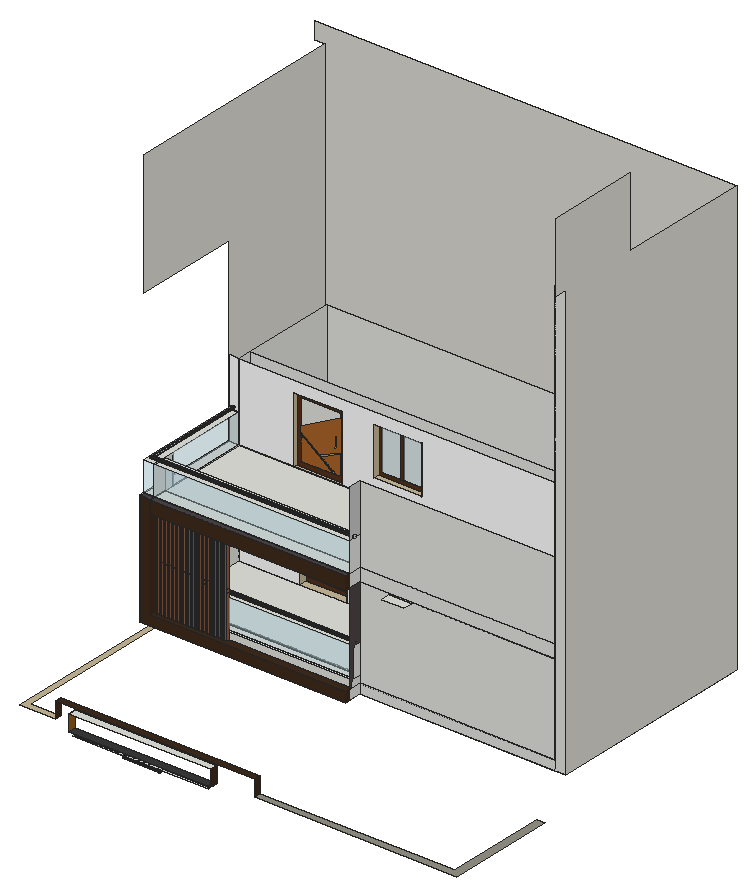
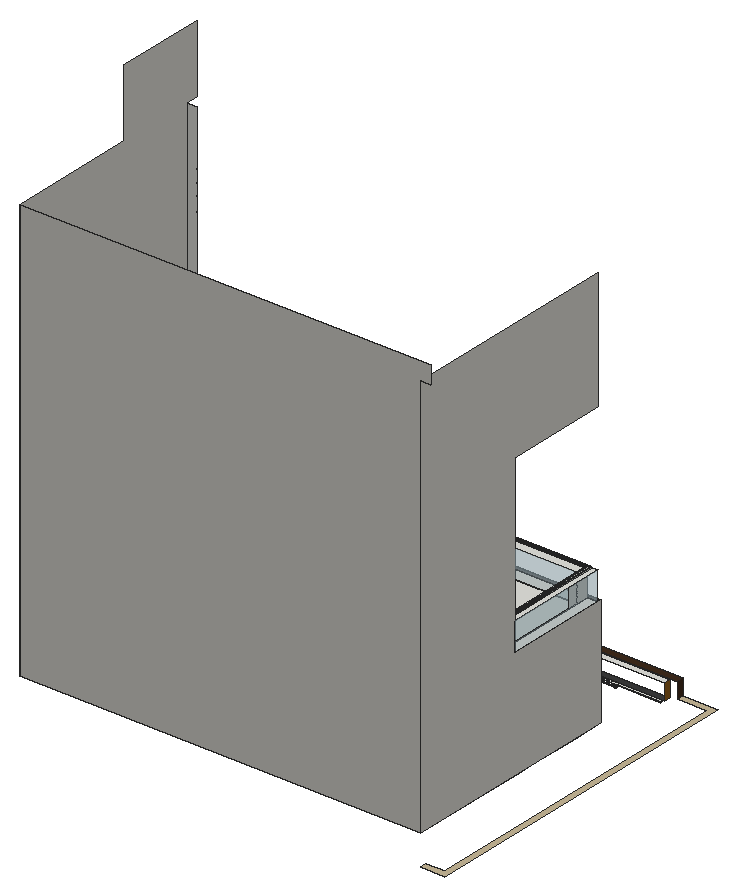
# SketchUp Ruby script. Lengths in inches.
U = 1.inch
M = Sketchup.active_model
def pt(a) = Geom::Point3d.new(a.map { |v| v * U })
def face(e, loops, mat)
  f = e.add_face(loops[0].map { |a| pt(a) })
  loops[1..].each { |l| e.add_face(l.map { |a| pt(a) }).erase! }
  f.material = f.back_material = mat if mat
  f
end
# faces: each face lists its corners as indices into pts; further lists are holes
def faces(e, pts, list, mat = nil) = list.each { |f| face(e, (f[0].is_a?(Array) ? f : [f]).map { |l| l.map { |i| pts[i] } }, mat) }
# xy, xz, yz: faces in a plane at the given z, y or x. An outline is a flat list of corners, or four numbers for a rectangle; further outlines are holes
def ring(l) = l.size == 4 ? [[l[0], l[1]], [l[2], l[1]], [l[2], l[3]], [l[0], l[3]]] : l.each_slice(2).to_a
def flat(e, list, mat, &to3) = list.each { |f| face(e, (f[0].is_a?(Array) ? f : [f]).map { |l| ring(l).map { |u, v| to3.(u, v) } }, mat) }
def xy(e, z, list, mat = nil) = flat(e, list, mat) { |x, y| [x, y, z] }
def xz(e, y, list, mat = nil) = flat(e, list, mat) { |x, z| [x, y, z] }
def yz(e, x, list, mat = nil) = flat(e, list, mat) { |y, z| [x, y, z] }
def lines(e, pts, list) = list.each { |a, b| e.add_line(pt(pts[a]), pt(pts[b])) }
# prism: a flat outline (further loops are holes) pulled along v
def prism(e, loops, v, mat = nil)
  f = face(e, loops, mat); d = Geom::Vector3d.new(v.map { |x| x * U })
  f.pushpull(f.normal.samedirection?(d) ? d.length : -d.length)
end
def box(e, o, s, mat = nil) = prism(e, [[o, [o[0] + s[0], o[1], o[2]], [o[0] + s[0], o[1] + s[1], o[2]], [o[0], o[1] + s[1], o[2]]]], [0, 0, s[2]], mat)
def at(x, y, z, deg = 0) = Geom::Transformation.translation(pt([x, y, z])) * Geom::Transformation.rotation(ORIGIN, Z_AXIS, deg.degrees)
def axes(o, x, y, z) = Geom::Transformation.new([*x, 0, *y, 0, *z, 0, *pt(o).to_a, 1])
def part(name) = M.definitions.add(name)
# library, detail: a bought-in or finely detailed component or shape, given as its bounding box
def library(name, o, s) = part(name).tap { |d| box(d.entities, o, s) }
def detail(e, o, s) = box(e.add_group.entities, o, s)
def put(e, d, t, mat = nil) = e.add_instance(d, t).tap { |i| i.material = mat if mat }
def group(e, t, mat = nil) = e.add_group.tap { |g| g.transformation = t; g.material = mat if mat }.entities
root = M.entities
M.materials.add("[Asphalt New]").color = [76, 68, 70]
M.materials.add("[Blinds Weave]").color = [141, 91, 25]
M.materials.add("[Carrera Marble]").color = [252, 252, 252]
M.materials.add("[Carrera Marble]1").color = [247, 247, 247]
M.materials.add("[Color M02]").color = [198, 198, 198]
M.materials.add("[Color M07]").color = [58, 58, 58]
M.materials.add("[Formica Graystone]1").color = [149, 146, 135]
M.materials.add("[Formica Speckled Grey]").color = [94, 105, 111]
M.materials.add("[Quartz Light Brown]").color = [199, 184, 152]
M.materials.add("[Quartz Light Grey]").color = [251, 251, 252]
M.materials.add("[Sandstone]").color = [63, 43, 28]
M.materials.add("[Terrazzo Tile Light]").color = [219, 217, 210]
M.materials.add("[Translucent Glass Safety]").color = [213, 245, 255]
M.materials["[Translucent Glass Safety]"].alpha = 0.35
M.materials.add("[Wood Bamboo]").color = [168, 99, 40]
M.materials.add("[Wood Floor Light]").color = [181, 156, 112]
M.materials.add("[Wood Veneer 01]").color = [84, 49, 25]
M.materials.add("[Wood Veneer 01]1").color = [120, 70, 37]
M.materials.add("[Wood Veneer 02]").color = [140, 94, 67]
xy(root,91.34,[[140.74,279.21,201.14,281.7],[201.14,279.21,204.61,288.34],[204.61,279.21,225.67,288.34],[229.25,279.21,232.82,288.34],[232.82,279.21,253.76,288.34],
  [253.76,279.21,256.89,288.34],[256.89,279.21,321.11,281.7],[140.74,281.7,201.14,286.88],[256.89,281.7,321.11,286.72],[256.89,286.72,321.11,288.34],
  [140.74,286.88,201.14,288.34]])
xy(root,94.91,[[136.3,279.21,319.42,288.34],[319.42,279.21,324.42,288.34]],"[Color M07]")
xy(root,103.14,[[381.67,279.21,649.65,279.21,649.65,424.96,639.83,424.96,639.83,288.34,381.67,288.34]],"[Formica Graystone]1")
xy(root,103.14,[[71.32,279.21,118.15,279.21,118.15,288.34,78.57,288.34,78.57,734.15,104.01,734.15,104.01,742.77,71.32,742.77]],"[Quartz Light Brown]")
xy(root,116.23,[[136.3,279.21,324.42,288.34]])
xy(root,124.77,[[118.15,279.21,324.42,288.34],[324.42,279.21,381.67,288.34]],"[Sandstone]")
xy(root,144.48,[[635.51,460.01,649.65,725.53],[104.01,479.96,118.15,505.27],[104.01,546.4,118.15,571.71],[104.01,614.47,118.15,639.78],[104.01,670,118.15,695.31],
  [104.01,725.53,118.15,742.77],[118.15,725.53,649.65,742.77]])
xy(root,144.48,[[104.01,436.33,104.01,479.96,118.15,479.96,118.15,505.27,104.01,505.27,104.01,546.4,118.15,546.4,118.15,571.71,104.01,571.71,104.01,614.47,118.15,614.47,118.15,639.78,104.01,639.78,104.01,670,118.15,670,118.15,695.31,104.01,695.31,104.01,725.53,635.51,725.53,635.51,460.01,376.83,460.01,376.83,436.33]],"[Carrera Marble]1")
xy(root,157.48,[[120.21,442.77,123.03,446.4],[125.53,442.77,128.34,446.4],[130.84,442.77,133.65,446.4],[136.15,442.77,138.96,446.4],[141.46,442.77,144.28,446.4],
  [146.78,442.77,149.59,446.4],[151.71,442.77,154.53,446.4],[156.65,442.77,159.46,446.4],[161.59,442.77,164.4,446.4],[166.53,442.77,169.34,446.4],
  [171.46,442.77,174.28,446.4],[176.4,442.77,179.21,446.4],[181.34,442.77,184.15,446.4],[186.28,442.77,189.09,446.4],[191.21,442.77,194.03,446.4],
  [196.15,442.77,198.96,446.4],[201.09,442.77,203.9,446.4],[206.03,442.77,208.84,446.4],[210.96,442.77,213.78,446.4],[118.15,447,376.83,460.01],
  [118.15,460.01,635.5,474.16],[118.15,474.16,635.5,583.41],[118.15,583.41,118.15,601.39,635.5,601.39,635.5,583.41,261.36,583.41,261.36,593.72,198.43,593.72,198.43,583.41],[118.15,601.39,635.5,728.625]])
xy(root,157.48,[[198.43,583.41,261.36,593.72]],"[Quartz Light Brown]")
xy(root,157.48,[[[118.15,436.33,376.83,447],[210.96,442.77,213.78,446.4],[206.03,442.77,208.84,446.4],[201.09,442.77,203.9,446.4],[196.15,442.77,198.96,446.4],[191.21,442.77,194.03,446.4],[186.28,442.77,189.09,446.4],[181.34,442.77,184.15,446.4],[176.4,442.77,179.21,446.4],[171.46,442.77,174.28,446.4],[166.53,442.77,169.34,446.4],[161.59,442.77,164.4,446.4],[156.65,442.77,159.46,446.4],[151.71,442.77,154.53,446.4],[146.78,442.77,149.59,446.4],[141.46,442.77,144.28,446.4],[136.15,442.77,138.96,446.4],[130.84,442.77,133.65,446.4],[125.53,442.77,128.34,446.4],[120.21,442.77,123.03,446.4]]],"[Sandstone]")
xy(root,166.35,[[118.15,449.94,376.83,460.01]])
xy(root,166.35,[[118.15,447,376.83,449.94]],"[Quartz Light Grey]")
xy(root,185.49,[[297.75,583.41,366.57,591.78]],"[Quartz Light Brown]")
xy(root,205.54,[[118.15,449.94,376.83,460.01]])
xy(root,259.32,[[198.43,583.41,261.36,593.72]],"[Quartz Light Brown]")
xy(root,261.87,[[297.75,583.41,366.57,591.78]],"[Quartz Light Brown]")
xy(root,277.48,[[118.15,583.41,635.5,601.39],[118.15,601.39,635.5,728.625]])
xy(root,277.48,[[[118.15,436.33,118.15,583.41,635.5,583.41,635.5,460.01,376.83,460.01,376.83,436.33],[151.71,442.77,154.53,446.4],[166.53,442.77,169.34,446.4],[176.4,442.77,179.21,446.4],[191.21,442.77,194.03,446.4],[201.09,442.77,203.9,446.4],[206.03,442.77,208.84,446.4],[210.96,442.77,213.78,446.4],[196.15,442.77,198.96,446.4],[186.28,442.77,189.09,446.4],[171.46,442.77,174.28,446.4],[181.34,442.77,184.15,446.4],[161.59,442.77,164.4,446.4],[156.65,442.77,159.46,446.4],[146.78,442.77,149.59,446.4],[141.46,442.77,144.28,446.4],[136.15,442.77,138.96,446.4],[125.53,442.77,128.34,446.4],[130.84,442.77,133.65,446.4],[120.21,442.77,123.03,446.4]]],"[Wood Veneer 01]1")
xy(root,278.96,[[419.27,442.77,449.02,455.21]])
xy(root,294.73,[[104.01,442.77,118.15,583.41],[118.15,442.77,376.83,460.01],[118.15,460.01,635.5,583.41],[118.15,583.41,118.15,601.39,635.5,601.39,635.5,583.41,253.72,583.41,253.72,588.28,190.84,588.28,190.84,583.41],[118.15,601.39,635.5,728.625]])
xy(root,294.73,[[104.01,436.33,118.15,442.77],[118.15,436.33,376.83,442.77]],"[Asphalt New]")
xy(root,294.73,[[190.84,583.41,253.72,588.28]],"[Quartz Light Brown]")
xy(root,318.08,[[295.95,583.41,360.57,591.84]],"[Quartz Light Brown]")
xy(root,333.73,[[104.01,442.77,118.15,583.41],[118.15,442.77,376.83,460.01]])
xz(root,436.33,[[104.01,144.48,376.83,144.48,376.83,157.48,118.15,157.48,118.15,294.73,104.01,294.73],[118.15,277.48,376.83,294.73]],"[Sandstone]")
xz(root,442.77,[[104.01,294.73,118.15,333.73],[118.15,294.73,376.83,333.73]],"[Translucent Glass Safety]")
xz(root,442.77,[[120.21,157.48,123.03,277.48],[125.53,157.48,128.34,277.48],[130.84,157.48,133.65,277.48],[136.15,157.48,138.96,277.48],[141.46,157.48,144.28,277.48],
  [146.78,157.48,149.59,277.48],[151.71,157.48,154.53,277.48],[156.65,157.48,159.46,277.48],[161.59,157.48,164.4,277.48],[166.53,157.48,169.34,277.48],
  [171.46,157.48,174.28,277.48],[176.4,157.48,179.21,277.48],[181.34,157.48,184.15,277.48],[186.28,157.48,189.09,277.48],[191.21,157.48,194.03,277.48],
  [196.15,157.48,198.96,277.48],[201.09,157.48,203.9,277.48],[206.03,157.48,208.84,277.48],[210.96,157.48,213.78,277.48]],"[Wood Veneer 02]")
xz(root,446.4,[[120.21,157.48,123.03,277.48],[125.53,157.48,128.34,277.48],[130.84,157.48,133.65,277.48],[136.15,157.48,138.96,277.48],[141.46,157.48,144.28,277.48],
  [146.78,157.48,149.59,277.48],[151.71,157.48,154.53,277.48],[156.65,157.48,159.46,277.48],[161.59,157.48,164.4,277.48],[166.53,157.48,169.34,277.48],
  [171.46,157.48,174.28,277.48],[176.4,157.48,179.21,277.48],[181.34,157.48,184.15,277.48],[186.28,157.48,189.09,277.48],[191.21,157.48,194.03,277.48],
  [196.15,157.48,198.96,277.48],[201.09,157.48,203.9,277.48],[206.03,157.48,208.84,277.48],[210.96,157.48,213.78,277.48]])
xz(root,447,[[118.15,157.48,376.83,166.35]])
xz(root,449.94,[[118.15,166.35,376.83,205.54]],"[Translucent Glass Safety]")
xz(root,460.01,[[376.83,144.48,376.83,157.48,635.5,157.48,635.5,719.42,635.51,719.42,635.51,144.48],[635.51,144.48,649.65,719.42],[118.15,157.48,376.83,166.35],[376.83,157.48,635.5,277.48],[376.83,277.48,635.5,294.73],
  [376.83,294.73,635.5,397.48]])
xz(root,460.01,[[118.15,166.35,376.83,205.54],[118.15,294.73,376.83,333.73]],"[Translucent Glass Safety]")
xz(root,583.41,[[118.15,277.48,635.5,294.73],[104.01,294.73,118.15,333.73],[110.36,335.3,109.91,335.36,109.49,335.54,109.125,335.82,108.85,336.18,108.67,336.6,108.61,337.05,108.67,337.51,108.85,337.93,109.125,338.29,109.49,338.57,109.91,338.74,110.36,338.8,110.82,338.74,111.24,338.57,111.6,338.29,111.88,337.93,112.05,337.51,112.11,337.05,112.05,336.6,111.88,336.18,111.6,335.82,111.24,335.54,110.82,335.36]])
xz(root,583.41,[[[118.15,157.48,198.43,157.48,198.43,259.32,261.36,259.32,261.36,157.48,635.5,157.48,635.5,277.48,118.15,277.48],[297.75,185.49,366.57,261.87]],[[118.15,294.73,190.84,294.73,190.84,382.42,253.72,382.42,253.72,294.73,635.5,294.73,635.5,397.48,118.15,397.48],[295.95,318.08,360.57,382.71]],[[104.01,333.73,118.15,397.48],[110.36,335.3,109.91,335.36,109.49,335.54,109.125,335.82,108.85,336.18,108.67,336.6,108.61,337.05,108.67,337.51,108.85,337.93,109.125,338.29,109.49,338.57,109.91,338.74,110.36,338.8,110.82,338.74,111.24,338.57,111.6,338.29,111.88,337.93,112.05,337.51,112.11,337.05,112.05,336.6,111.88,336.18,111.6,335.82,111.24,335.54,110.82,335.36]]],"[Carrera Marble]")
xz(root,588.28,[[196.19,300.08,239.31,300.08,196.19,333.54],[243.83,300.08,248.36,300.08,248.36,328.05,223.1,315.82],[[221.41,317.11,248.36,329.54,248.36,370.39,196.19,342.9,196.19,336.25],[241.46,332.55,244.09,347.42]]],"[Wood Bamboo]")
xz(root,588.28,[[239.31,300.08,243.83,300.08,223.1,315.82,221.41,317.11,196.19,336.25,196.19,333.54],[223.1,315.82,248.36,328.05,248.36,329.54,221.41,317.11],[241.46,332.55,244.09,347.42]],"[Wood Floor Light]")
xz(root,588.28,[[[190.84,294.73,253.72,382.42],[196.19,300.08,248.36,377.07]]],"[Wood Veneer 01]")
xz(root,591.78,[[302.4,190.14,329.66,257.22],[333.51,190.14,361.92,257.22]],"[Translucent Glass Safety]")
xz(root,591.78,[[[297.75,185.49,366.57,261.87],[302.4,190.14,361.92,257.22]],[329.66,190.14,333.51,257.22]],"[Wood Veneer 01]")
xz(root,591.84,[[300.36,322.5,326.01,378.29],[330.23,322.5,356.16,378.29]],"[Translucent Glass Safety]")
xz(root,591.84,[[[295.95,318.08,360.57,382.71],[300.36,322.5,356.16,378.29]],[326.01,322.5,330.23,378.29]],"[Wood Veneer 01]")
xz(root,593.72,[[203.53,162.59,238.88,162.59,203.53,197.93],[242.05,162.59,256.26,162.59,256.26,187.54,231.08,173.5625],[[228.95,175.6875,256.26,190.75,256.26,244.96,203.53,212.24,203.53,201.1],[248.32,199.43,252.13,217.87]],[203.53,215.39,245.22,240.77,203.53,247.49],[246.7,241.67,256.26,247.49,256.26,254.21,203.53,254.21,203.53,249.42]],"[Wood Bamboo]")
xz(root,593.72,[[238.88,162.59,242.05,162.59,231.08,173.5625,228.95,175.6875,203.53,201.1,203.53,197.93],[231.08,173.5625,256.26,187.54,256.26,190.75,228.95,175.6875],[248.32,199.43,252.13,217.87],[203.53,212.24,256.26,244.96,256.26,247.49,246.7,241.67,245.22,240.77,203.53,215.39],[245.22,240.77,246.7,241.67,203.53,249.42,203.53,247.49]],"[Wood Floor Light]")
xz(root,593.72,[[[198.43,157.48,261.36,259.32],[203.53,162.59,256.26,254.21]]],"[Wood Veneer 01]")
xz(root,601.39,[[118.15,157.48,635.5,277.48],[118.15,277.48,635.5,294.73],[118.15,294.73,635.5,397.48]])
xz(root,728.625,[[118.15,157.48,635.5,277.48],[118.15,277.48,635.5,294.73],[118.15,294.73,635.5,397.48]])
xz(root,742.77,[[104.01,144.48,104.01,695.82,91.26,695.82,91.26,719.42,649.65,719.42,649.65,144.48]],"[Terrazzo Tile Light]")
yz(root,104.01,[[436.33,144.48,436.33,294.73,583.41,294.73,583.41,532.23,442.77,532.23,442.77,695.82,742.77,695.82,742.77,144.48]],"[Terrazzo Tile Light]")
yz(root,104.01,[[442.77,294.73,583.41,333.73]],"[Translucent Glass Safety]")
yz(root,118.15,[[447,157.48,460.01,166.35],[474.16,157.48,583.41,277.48],[583.41,157.48,601.39,277.48],[601.39,157.48,728.625,277.48],[449.94,166.35,460.01,205.54],
  [436.33,277.48,460.01,294.73],[460.01,277.48,474.16,294.73],[474.16,277.48,583.41,294.73],[583.41,277.48,601.39,294.73],[601.39,277.48,728.625,294.73],
  [442.77,294.73,460.01,333.73],[460.01,294.73,474.16,333.73],[583.41,294.73,601.39,397.48],[601.39,294.73,728.625,397.48]])
yz(root,118.15,[[279.21,103.14,288.34,124.77],[[436.33,157.48,447,157.48,447,166.35,449.94,166.35,449.94,205.54,460.01,205.54,460.01,157.48,474.16,157.48,474.16,277.48,436.33,277.48],[453.83,207.59,453.36,207.66,452.92,207.84,452.55,208.125,452.26,208.5,452.08,208.9375,452.02,209.41,452.08,209.875,452.26,210.3125,452.55,210.6875,452.92,210.98,453.36,211.16,453.83,211.22,454.3,211.16,454.74,210.98,455.11,210.6875,455.4,210.3125,455.58,209.875,455.64,209.41,455.58,208.9375,455.4,208.5,455.11,208.125,454.74,207.84,454.3,207.66]]],"[Sandstone]")
yz(root,118.15,[[474.16,294.73,583.41,333.73]],"[Translucent Glass Safety]")
yz(root,120.21,[[442.77,157.48,446.4,277.48]],"[Wood Veneer 02]")
yz(root,123.03,[[442.77,157.48,446.4,277.48]],"[Wood Veneer 02]")
yz(root,125.53,[[442.77,157.48,446.4,277.48]],"[Wood Veneer 02]")
yz(root,128.34,[[442.77,157.48,446.4,277.48]],"[Wood Veneer 02]")
yz(root,130.84,[[442.77,157.48,446.4,277.48]],"[Wood Veneer 02]")
yz(root,133.65,[[442.77,157.48,446.4,277.48]],"[Wood Veneer 02]")
yz(root,136.15,[[442.77,157.48,446.4,277.48]],"[Wood Veneer 02]")
yz(root,136.3,[[279.21,94.91,288.34,116.23]],"[Blinds Weave]")
yz(root,138.96,[[442.77,157.48,446.4,277.48]],"[Wood Veneer 02]")
yz(root,141.46,[[442.77,157.48,446.4,277.48]],"[Wood Veneer 02]")
yz(root,144.28,[[442.77,157.48,446.4,277.48]],"[Wood Veneer 02]")
yz(root,146.78,[[442.77,157.48,446.4,277.48]],"[Wood Veneer 02]")
yz(root,149.59,[[442.77,157.48,446.4,277.48]],"[Wood Veneer 02]")
yz(root,151.71,[[442.77,157.48,446.4,277.48]],"[Wood Veneer 02]")
yz(root,154.53,[[442.77,157.48,446.4,277.48]],"[Wood Veneer 02]")
yz(root,156.65,[[442.77,157.48,446.4,277.48]],"[Wood Veneer 02]")
yz(root,159.46,[[442.77,157.48,446.4,277.48]],"[Wood Veneer 02]")
yz(root,161.59,[[442.77,157.48,446.4,277.48]],"[Wood Veneer 02]")
yz(root,164.4,[[442.77,157.48,446.4,277.48]],"[Wood Veneer 02]")
yz(root,166.53,[[442.77,157.48,446.4,277.48]],"[Wood Veneer 02]")
yz(root,169.34,[[442.77,157.48,446.4,277.48]],"[Wood Veneer 02]")
yz(root,171.46,[[442.77,157.48,446.4,277.48]],"[Wood Veneer 02]")
yz(root,174.28,[[442.77,157.48,446.4,277.48]],"[Wood Veneer 02]")
yz(root,176.4,[[442.77,157.48,446.4,277.48]],"[Wood Veneer 02]")
yz(root,179.21,[[442.77,157.48,446.4,277.48]],"[Wood Veneer 02]")
yz(root,181.34,[[442.77,157.48,446.4,277.48]],"[Wood Veneer 02]")
yz(root,184.15,[[442.77,157.48,446.4,277.48]],"[Wood Veneer 02]")
yz(root,186.28,[[442.77,157.48,446.4,277.48]],"[Wood Veneer 02]")
yz(root,189.09,[[442.77,157.48,446.4,277.48]],"[Wood Veneer 02]")
yz(root,190.84,[[583.41,294.73,588.28,382.42]],"[Quartz Light Brown]")
yz(root,191.21,[[442.77,157.48,446.4,277.48]],"[Wood Veneer 02]")
yz(root,194.03,[[442.77,157.48,446.4,277.48]],"[Wood Veneer 02]")
yz(root,196.15,[[442.77,157.48,446.4,277.48]],"[Wood Veneer 02]")
yz(root,198.43,[[583.41,157.48,593.72,259.32]],"[Quartz Light Brown]")
yz(root,198.96,[[442.77,157.48,446.4,277.48]],"[Wood Veneer 02]")
yz(root,201.09,[[442.77,157.48,446.4,277.48]],"[Wood Veneer 02]")
yz(root,203.9,[[442.77,157.48,446.4,277.48]],"[Wood Veneer 02]")
yz(root,204.61,[[283.74,84.95,283.58,84.97,283.43,85.03,283.3,85.13,283.2,85.26,283.14,85.41,283.12,85.57,283.14,85.73,283.2,85.88,283.3,86.01,283.43,86.11,283.58,86.18,283.74,86.2,283.9,86.18,284.05,86.11,284.18,86.01,284.28,85.88,284.34,85.73,284.37,85.57,284.34,85.41,284.28,85.26,284.18,85.13,284.05,85.03,283.9,84.97],[283.74,87.76,283.58,87.78,283.43,87.84,283.3,87.94,283.2,88.07,283.14,88.22,283.12,88.38,283.14,88.55,283.2,88.7,283.3,88.83,283.43,88.93,283.58,88.99,283.74,89.01,283.9,88.99,284.05,88.93,284.18,88.83,284.28,88.7,284.34,88.55,284.37,88.38,284.34,88.22,284.28,88.07,284.18,87.94,284.05,87.84,283.9,87.78]])
yz(root,206.03,[[442.77,157.48,446.4,277.48]],"[Wood Veneer 02]")
yz(root,208.84,[[442.77,157.48,446.4,277.48]],"[Wood Veneer 02]")
yz(root,210.96,[[442.77,157.48,446.4,277.48]],"[Wood Veneer 02]")
yz(root,213.78,[[442.77,157.48,446.4,277.48]],"[Wood Veneer 02]")
yz(root,253.72,[[583.41,294.73,588.28,382.42]],"[Quartz Light Brown]")
yz(root,261.36,[[583.41,157.48,593.72,259.32]],"[Quartz Light Brown]")
yz(root,295.95,[[583.41,318.08,591.84,382.71]],"[Quartz Light Brown]")
yz(root,297.75,[[583.41,185.49,591.78,261.87]],"[Quartz Light Brown]")
yz(root,324.42,[[279.21,94.91,288.34,116.23]],"[Sandstone]")
yz(root,360.57,[[583.41,318.08,591.84,382.71]],"[Quartz Light Brown]")
yz(root,366.57,[[583.41,185.49,591.78,261.87]],"[Quartz Light Brown]")
yz(root,376.83,[[442.77,144.48,460.01,157.48],[447,157.48,460.01,166.35],[449.94,166.35,460.01,205.54],[453.83,207.59,454.3,207.66,454.74,207.84,455.11,208.125,455.4,208.5,455.58,208.9375,455.64,209.41,455.58,209.875,455.4,210.3125,455.11,210.6875,454.74,210.98,454.3,211.16,453.83,211.22,453.36,211.16,452.92,210.98,452.55,210.6875,452.26,210.3125,452.08,209.875,452.02,209.41,452.08,208.9375,452.26,208.5,452.55,208.125,452.92,207.84,453.36,207.66],[442.77,277.48,460.01,294.73],
  [442.77,294.73,460.01,333.73]])
yz(root,376.83,[[[442.77,157.48,442.77,277.48,460.01,277.48,460.01,205.54,449.94,205.54,449.94,166.35,447,166.35,447,157.48],[453.83,207.59,454.3,207.66,454.74,207.84,455.11,208.125,455.4,208.5,455.58,208.9375,455.64,209.41,455.58,209.875,455.4,210.3125,455.11,210.6875,454.74,210.98,454.3,211.16,453.83,211.22,453.36,211.16,452.92,210.98,452.55,210.6875,452.26,210.3125,452.08,209.875,452.02,209.41,452.08,208.9375,452.26,208.5,452.55,208.125,452.92,207.84,453.36,207.66]]],"[Asphalt New]")
yz(root,376.83,[[442.77,333.73,460.01,397.48]],"[Color M02]")
yz(root,376.83,[[436.33,144.48,442.77,157.48],[436.33,277.48,442.77,294.73]],"[Sandstone]")
yz(root,379.18,[[448.91,335.3,449.36,335.36,449.78,335.54,450.14,335.82,450.42,336.18,450.6,336.6,450.66,337.05,450.6,337.51,450.42,337.93,450.14,338.29,449.78,338.57,449.36,338.74,448.91,338.8,448.45,338.74,448.03,338.57,447.67,338.29,447.39,337.93,447.22,337.51,447.16,337.05,447.22,336.6,447.39,336.18,447.67,335.82,448.03,335.54,448.45,335.36]])
yz(root,381.67,[[279.21,103.14,288.34,124.77]],"[Sandstone]")
yz(root,635.5,[[460.01,157.48,474.16,277.48],[583.41,157.48,601.39,277.48],[601.39,157.48,728.625,277.48],[460.01,277.48,474.16,294.73],[474.16,277.48,583.41,294.73],
  [583.41,277.48,601.39,294.73],[601.39,277.48,728.625,294.73],[460.01,294.73,474.16,397.48],[583.41,294.73,601.39,397.48],[601.39,294.73,728.625,397.48]])
yz(root,635.5,[[474.16,157.48,583.41,277.48],[474.16,294.73,583.41,397.48]],"[Carrera Marble]")
yz(root,649.65,[[460.01,144.48,742.77,144.48,742.77,719.42,566.02,719.42,566.02,812.1,442.77,812.1,442.77,719.42,460.01,719.42]],"[Terrazzo Tile Light]")
p = [[204.61,283.58,84.97],[204.61,283.74,84.95],[253.76,283.74,84.95],[253.76,283.58,84.97],[204.61,283.9,84.97],[253.76,283.9,84.97],
  [204.61,283.3,85.13],[204.61,283.43,85.03],[253.76,283.43,85.03],[253.76,283.3,85.13],[204.61,284.05,85.03],[253.76,284.05,85.03],
  [204.61,284.18,85.13],[253.76,284.18,85.13],[204.61,283.2,85.26],[253.76,283.2,85.26],[204.61,284.28,85.26],[253.76,284.28,85.26],
  [204.61,283.14,85.41],[253.76,283.14,85.41],[204.61,284.34,85.41],[253.76,284.34,85.41],[204.61,283.12,85.57],[253.76,283.12,85.57],
  [204.61,284.37,85.57],[253.76,284.37,85.57],[204.61,283.14,85.73],[253.76,283.14,85.73],[204.61,284.34,85.73],[253.76,284.34,85.73],
  [204.61,283.2,85.88],[253.76,283.2,85.88],[204.61,284.28,85.88],[253.76,284.28,85.88],[204.61,283.3,86.01],[253.76,283.3,86.01],
  [204.61,284.18,86.01],[253.76,284.18,86.01],[204.61,283.43,86.11],[253.76,283.43,86.11],[204.61,284.05,86.11],[253.76,284.05,86.11],
  [204.61,283.58,86.18],[253.76,283.58,86.18],[204.61,283.9,86.18],[253.76,283.9,86.18],[204.61,283.74,86.2],[253.76,283.74,86.2],
  [204.61,283.3,87.94],[204.61,283.43,87.84],[253.76,283.43,87.84],[253.76,283.3,87.94],[204.61,283.58,87.78],[253.76,283.58,87.78],
  [204.61,283.74,87.76],[253.76,283.74,87.76],[204.61,283.9,87.78],[253.76,283.9,87.78],[204.61,284.05,87.84],[253.76,284.05,87.84],
  [204.61,284.18,87.94],[253.76,284.18,87.94],[204.61,283.2,88.07],[253.76,283.2,88.07],[204.61,284.28,88.07],[253.76,284.28,88.07],
  [204.61,283.14,88.22],[253.76,283.14,88.22],[204.61,284.34,88.22],[253.76,284.34,88.22],[204.61,283.12,88.38],[253.76,283.12,88.38],
  [204.61,284.37,88.38],[253.76,284.37,88.38],[204.61,283.14,88.55],[253.76,283.14,88.55],[204.61,284.34,88.55],[253.76,284.34,88.55],
  [204.61,283.2,88.7],[253.76,283.2,88.7],[204.61,284.28,88.7],[253.76,284.28,88.7],[204.61,283.3,88.83],[253.76,283.3,88.83],
  [204.61,284.18,88.83],[253.76,284.18,88.83],[204.61,283.43,88.93],[253.76,283.43,88.93],[204.61,284.05,88.93],[253.76,284.05,88.93],
  [204.61,283.58,88.99],[253.76,283.58,88.99],[204.61,283.9,88.99],[253.76,283.9,88.99],[204.61,283.74,89.01],[253.76,283.74,89.01],
  [376.83,453.83,207.59],[376.83,453.36,207.66],[118.15,453.36,207.66],[118.15,453.83,207.59],[376.83,454.3,207.66],[118.15,454.3,207.66],
  [376.83,452.92,207.84],[118.15,452.92,207.84],[376.83,454.74,207.84],[118.15,454.74,207.84],[376.83,452.55,208.125],[118.15,452.55,208.125],
  [376.83,455.11,208.125],[118.15,455.11,208.125],[376.83,452.26,208.5],[118.15,452.26,208.5],[376.83,455.4,208.5],[118.15,455.4,208.5],
  [376.83,452.08,208.9375],[118.15,452.08,208.9375],[376.83,455.58,208.9375],[118.15,455.58,208.9375],[376.83,452.02,209.41],[118.15,452.02,209.41],
  [376.83,455.64,209.41],[118.15,455.64,209.41],[376.83,452.08,209.875],[118.15,452.08,209.875],[376.83,455.58,209.875],[118.15,455.58,209.875],
  [376.83,452.26,210.3125],[118.15,452.26,210.3125],[376.83,455.4,210.3125],[118.15,455.4,210.3125],[376.83,452.55,210.6875],[118.15,452.55,210.6875],
  [376.83,455.11,210.6875],[118.15,455.11,210.6875],[376.83,452.92,210.98],[118.15,452.92,210.98],[376.83,454.74,210.98],[118.15,454.74,210.98],
  [376.83,453.36,211.16],[118.15,453.36,211.16],[376.83,454.3,211.16],[118.15,454.3,211.16],[376.83,453.83,211.22],[118.15,453.83,211.22],
  [109.91,583.41,335.36],[110.36,583.41,335.3],[110.36,448.91,335.3],[109.91,448.45,335.36],[379.18,448.91,335.3],[379.18,448.45,335.36],
  [110.82,583.41,335.36],[110.82,449.36,335.36],[379.18,449.36,335.36],[109.49,583.41,335.54],[109.49,448.03,335.54],[379.18,448.03,335.54],
  [111.24,583.41,335.54],[111.24,449.78,335.54],[379.18,449.78,335.54],[109.125,583.41,335.82],[109.125,447.67,335.82],[379.18,447.67,335.82],
  [111.6,583.41,335.82],[111.6,450.14,335.82],[379.18,450.14,335.82],[108.85,583.41,336.18],[108.85,447.39,336.18],[379.18,447.39,336.18],
  [111.88,583.41,336.18],[111.88,450.42,336.18],[379.18,450.42,336.18],[108.67,583.41,336.6],[108.67,447.22,336.6],[379.18,447.22,336.6],
  [112.05,583.41,336.6],[112.05,450.6,336.6],[379.18,450.6,336.6],[108.61,583.41,337.05],[108.61,447.16,337.05],[379.18,447.16,337.05],
  [112.11,583.41,337.05],[112.11,450.66,337.05],[379.18,450.66,337.05],[108.67,583.41,337.51],[108.67,447.22,337.51],[379.18,447.22,337.51],
  [112.05,583.41,337.51],[112.05,450.6,337.51],[379.18,450.6,337.51],[108.85,583.41,337.93],[108.85,447.39,337.93],[379.18,447.39,337.93],
  [111.88,583.41,337.93],[111.88,450.42,337.93],[379.18,450.42,337.93],[109.125,583.41,338.29],[109.125,447.67,338.29],[379.18,447.67,338.29],
  [111.6,583.41,338.29],[111.6,450.14,338.29],[379.18,450.14,338.29],[109.49,583.41,338.57],[109.49,448.03,338.57],[379.18,448.03,338.57],
  [111.24,583.41,338.57],[111.24,449.78,338.57],[379.18,449.78,338.57],[109.91,583.41,338.74],[109.91,448.45,338.74],[379.18,448.45,338.74],
  [110.82,583.41,338.74],[110.82,449.36,338.74],[379.18,449.36,338.74],[110.36,583.41,338.8],[110.36,448.91,338.8],[379.18,448.91,338.8],
  [110.36,583.41,337.05],[110.36,448.91,337.05],[379.18,448.91,337.05]]
faces(root,p,[[0,1,2,3],[1,4,5,2],[6,7,8,9],[7,0,3,8],[4,10,11,5],[10,12,13,11],[14,6,9,15],[12,16,17,13],
  [18,14,15,19],[16,20,21,17],[22,18,19,23],[20,24,25,21],[26,22,23,27],[24,28,29,25],[30,26,27,31],[28,32,33,29],
  [34,30,31,35],[32,36,37,33],[38,34,35,39],[36,40,41,37],[42,38,39,43],[40,44,45,41],[46,42,43,47],[44,46,47,45],
  [48,49,50,51],[49,52,53,50],[52,54,55,53],[54,56,57,55],[56,58,59,57],[58,60,61,59],[62,48,51,63],[60,64,65,61],
  [66,62,63,67],[64,68,69,65],[70,66,67,71],[68,72,73,69],[74,70,71,75],[72,76,77,73],[78,74,75,79],[76,80,81,77],
  [82,78,79,83],[80,84,85,81],[86,82,83,87],[84,88,89,85],[90,86,87,91],[88,92,93,89],[94,90,91,95],[92,94,95,93]],"[Formica Speckled Grey]")
faces(root,p,[[96,97,98,99],[100,96,99,101],[97,102,103,98],[104,100,101,105],[102,106,107,103],[108,104,105,109],[106,110,111,107],[112,108,109,113],
  [110,114,115,111],[116,112,113,117],[114,118,119,115],[120,116,117,121],[118,122,123,119],[124,120,121,125],[122,126,127,123],[128,124,125,129],
  [126,130,131,127],[132,128,129,133],[130,134,135,131],[136,132,133,137],[134,138,139,135],[140,136,137,141],[138,142,143,139],[142,140,141,143],
  [144,145,146,147],[147,146,148,149],[145,150,151,146],[146,151,152,148],[153,144,147,154],[154,147,149,155],[150,156,157,151],[151,157,158,152],
  [159,153,154,160],[160,154,155,161],[156,162,163,157],[157,163,164,158],[165,159,160,166],[166,160,161,167],[162,168,169,163],[163,169,170,164],
  [171,165,166,172],[172,166,167,173],[168,174,175,169],[169,175,176,170],[177,171,172,178],[178,172,173,179],[174,180,181,175],[175,181,182,176],
  [183,177,178,184],[184,178,179,185],[180,186,187,181],[181,187,188,182],[189,183,184,190],[190,184,185,191],[186,192,193,187],[187,193,194,188],
  [195,189,190,196],[196,190,191,197],[192,198,199,193],[193,199,200,194],[201,195,196,202],[202,196,197,203],[198,204,205,199],[199,205,206,200],
  [207,201,202,208],[208,202,203,209],[204,210,211,205],[205,211,212,206],[213,207,208,214],[214,208,209,215],[210,213,214,211],[211,214,215,212]],"[Terrazzo Tile Light]")
lines(root,p,[[216,217],[217,218]])
